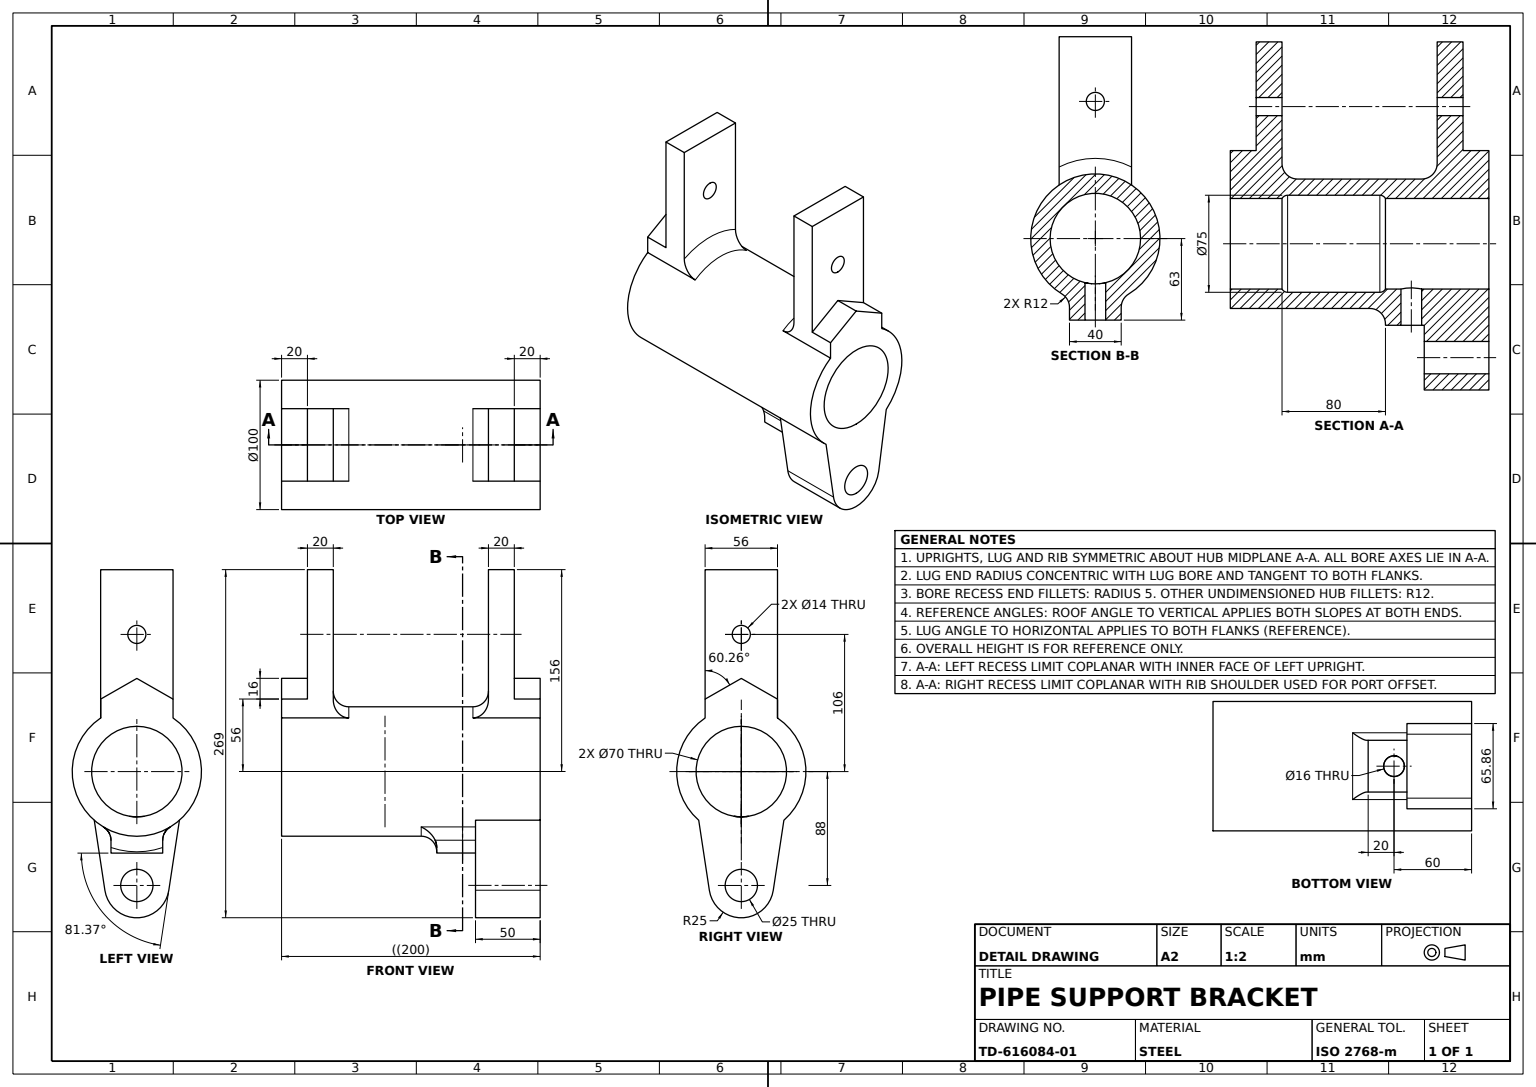
ISO-10303-21;
HEADER;
FILE_DESCRIPTION((''),'2;1');
FILE_NAME('','',(''),(''),'','','');
FILE_SCHEMA(('AUTOMOTIVE_DESIGN'));
ENDSEC;
DATA;
#1=APPLICATION_CONTEXT('');
#2=PRODUCT_CONTEXT('',#1,'mechanical');
#3=PRODUCT('','','',(#2));
#4=PRODUCT_DEFINITION_FORMATION('','',#3);
#5=PRODUCT_DEFINITION_CONTEXT('',#1,'design');
#6=PRODUCT_DEFINITION('','',#4,#5);
#7=PRODUCT_DEFINITION_SHAPE('','',#6);
#8=(LENGTH_UNIT()NAMED_UNIT(*)SI_UNIT(.MILLI.,.METRE.));
#9=(NAMED_UNIT(*)PLANE_ANGLE_UNIT()SI_UNIT($,.RADIAN.));
#10=(NAMED_UNIT(*)SI_UNIT($,.STERADIAN.)SOLID_ANGLE_UNIT());
#11=UNCERTAINTY_MEASURE_WITH_UNIT(LENGTH_MEASURE(0.005),#8,'distance_accuracy_value','');
#12=(GEOMETRIC_REPRESENTATION_CONTEXT(3)GLOBAL_UNCERTAINTY_ASSIGNED_CONTEXT((#11))GLOBAL_UNIT_ASSIGNED_CONTEXT((#8,#9,#10))REPRESENTATION_CONTEXT('',''));
#13=CARTESIAN_POINT('',(-28.,-80.,156.));
#14=VERTEX_POINT('',#13);
#15=CARTESIAN_POINT('',(28.,-80.,156.));
#16=VERTEX_POINT('',#15);
#17=DIRECTION('',(1.,0.,0.));
#18=VECTOR('',#17,1000.);
#19=LINE('',#13,#18);
#20=EDGE_CURVE('',#14,#16,#19,.T.);
#21=ORIENTED_EDGE('',*,*,#20,.T.);
#22=CARTESIAN_POINT('',(28.,-60.,156.));
#23=VERTEX_POINT('',#22);
#24=DIRECTION('',(0.,-1.,0.));
#25=VECTOR('',#24,1000.);
#26=LINE('',#22,#25);
#27=EDGE_CURVE('',#23,#16,#26,.T.);
#28=ORIENTED_EDGE('',*,*,#27,.F.);
#29=CARTESIAN_POINT('',(-28.,-60.,156.));
#30=VERTEX_POINT('',#29);
#31=LINE('',#29,#18);
#32=EDGE_CURVE('',#30,#23,#31,.T.);
#33=ORIENTED_EDGE('',*,*,#32,.F.);
#34=LINE('',#29,#25);
#35=EDGE_CURVE('',#30,#14,#34,.T.);
#36=ORIENTED_EDGE('',*,*,#35,.T.);
#37=EDGE_LOOP('',(#21,#28,#33,#36));
#38=FACE_BOUND('',#37,.T.);
#39=DIRECTION('',(0.,0.,-1.));
#40=DIRECTION('',(-1.,0.,0.));
#41=AXIS2_PLACEMENT_3D('',#29,#39,#40);
#42=PLANE('',#41);
#43=ADVANCED_FACE('',(#38),#42,.F.);
#44=CARTESIAN_POINT('',(0.,-80.,113.));
#45=VERTEX_POINT('',#44);
#46=CARTESIAN_POINT('',(0.,-80.,106.));
#47=DIRECTION('',(0.,1.,0.));
#48=DIRECTION('',(0.,0.,1.));
#49=AXIS2_PLACEMENT_3D('',#46,#47,#48);
#50=CIRCLE('',#49,7.);
#51=EDGE_CURVE('',#45,#45,#50,.T.);
#52=ORIENTED_EDGE('',*,*,#51,.F.);
#53=EDGE_LOOP('',(#52));
#54=FACE_BOUND('',#53,.T.);
#55=CARTESIAN_POINT('',(0.,-60.,113.));
#56=VERTEX_POINT('',#55);
#57=CARTESIAN_POINT('',(0.,-60.,106.));
#58=AXIS2_PLACEMENT_3D('',#57,#47,#48);
#59=CIRCLE('',#58,7.);
#60=EDGE_CURVE('',#56,#56,#59,.T.);
#61=ORIENTED_EDGE('',*,*,#60,.T.);
#62=EDGE_LOOP('',(#61));
#63=FACE_BOUND('',#62,.T.);
#64=CARTESIAN_POINT('',(0.,80.,106.));
#65=AXIS2_PLACEMENT_3D('',#64,#24,#39);
#66=CYLINDRICAL_SURFACE('',#65,7.);
#67=ADVANCED_FACE('',(#54,#63),#66,.F.);
#68=CARTESIAN_POINT('',(0.,-55.669873,-37.5));
#69=VERTEX_POINT('',#68);
#70=CARTESIAN_POINT('',(0.,-55.669873,0.));
#71=AXIS2_PLACEMENT_3D('',#70,#24,#39);
#72=CIRCLE('',#71,37.5);
#73=EDGE_CURVE('',#69,#69,#72,.F.);
#74=ORIENTED_EDGE('',*,*,#73,.T.);
#75=EDGE_LOOP('',(#74));
#76=FACE_BOUND('',#75,.T.);
#77=CARTESIAN_POINT('',(0.,-60.,-35.));
#78=VERTEX_POINT('',#77);
#79=CARTESIAN_POINT('',(0.,-60.,0.));
#80=AXIS2_PLACEMENT_3D('',#79,#24,#39);
#81=CIRCLE('',#80,35.);
#82=EDGE_CURVE('',#78,#78,#81,.F.);
#83=ORIENTED_EDGE('',*,*,#82,.F.);
#84=EDGE_LOOP('',(#83));
#85=FACE_BOUND('',#84,.T.);
#86=TOROIDAL_SURFACE('',#71,32.5,5.);
#87=ADVANCED_FACE('',(#76,#85),#86,.F.);
#88=CARTESIAN_POINT('',(0.,20.,-35.));
#89=VERTEX_POINT('',#88);
#90=CARTESIAN_POINT('',(0.,20.,0.));
#91=AXIS2_PLACEMENT_3D('',#90,#24,#39);
#92=CIRCLE('',#91,35.);
#93=EDGE_CURVE('',#89,#89,#92,.F.);
#94=ORIENTED_EDGE('',*,*,#93,.F.);
#95=EDGE_LOOP('',(#94));
#96=FACE_BOUND('',#95,.T.);
#97=CARTESIAN_POINT('',(8.,40.,-34.07345));
#98=VERTEX_POINT('',#97);
#99=CARTESIAN_POINT('',(7.575345,43.162099,-34.177167));
#100=CARTESIAN_POINT('',(8.211573,39.997592,-34.021762));
#101=CARTESIAN_POINT('',(7.578363,36.847533,-34.176486));
#102=CARTESIAN_POINT('',(5.801674,34.196418,-34.54076));
#103=CARTESIAN_POINT('',(3.152048,32.421651,-34.900124));
#104=CARTESIAN_POINT('',(0.005682,31.79015,-35.049729));
#105=CARTESIAN_POINT('',(-3.145527,32.417757,-34.900958));
#106=CARTESIAN_POINT('',(-5.803296,34.197129,-34.540575));
#107=CARTESIAN_POINT('',(-7.579059,36.849247,-34.176286));
#108=CARTESIAN_POINT('',(-8.20982,39.996413,-34.022177));
#109=CARTESIAN_POINT('',(-7.581658,43.144978,-34.175707));
#110=CARTESIAN_POINT('',(-5.807641,45.797608,-34.539704));
#111=CARTESIAN_POINT('',(-3.157808,47.576789,-34.899734));
#112=CARTESIAN_POINT('',(-0.004516,48.210487,-35.049891));
#113=CARTESIAN_POINT('',(3.146995,47.581253,-34.9007));
#114=CARTESIAN_POINT('',(5.799133,45.805003,-34.541192));
#115=B_SPLINE_CURVE_WITH_KNOTS('',3,(#99,#100,#101,#102,#103,#104,#105,#106,#107,#108,#109,#110,#111,#112,#113,#114,#99,#100,#101),.UNSPECIFIED.,.T.,.F.,(1,1,1,1,1,1,1,1,1,1,1,1,1,1,1,1,1,1,1,1,1,1,1),(-0.009409243,-0.006272829,-0.003136414,0.,0.003136414,0.006272829,0.009409243,0.012545657,0.015682072,0.018818486,0.0219549,0.025091314,0.028227729,0.031364143,0.034500557,0.037636972,0.040773386,0.0439098,0.047046215,0.050182629,0.053319043,0.056455457,0.059591872),.UNSPECIFIED.);
#116=EDGE_CURVE('',#98,#98,#115,.T.);
#117=ORIENTED_EDGE('',*,*,#116,.T.);
#118=EDGE_LOOP('',(#117));
#119=FACE_BOUND('',#118,.T.);
#120=CARTESIAN_POINT('',(0.,100.,-35.));
#121=VERTEX_POINT('',#120);
#122=CARTESIAN_POINT('',(0.,100.,0.));
#123=AXIS2_PLACEMENT_3D('',#122,#24,#39);
#124=CIRCLE('',#123,35.);
#125=EDGE_CURVE('',#121,#121,#124,.T.);
#126=ORIENTED_EDGE('',*,*,#125,.F.);
#127=EDGE_LOOP('',(#126));
#128=FACE_BOUND('',#127,.T.);
#129=CARTESIAN_POINT('',(0.,-100.,0.));
#130=AXIS2_PLACEMENT_3D('',#129,#47,#48);
#131=CYLINDRICAL_SURFACE('',#130,35.);
#132=ADVANCED_FACE('',(#96,#119,#128),#131,.F.);
#133=CARTESIAN_POINT('',(-28.,60.,156.));
#134=VERTEX_POINT('',#133);
#135=CARTESIAN_POINT('',(-28.,80.,156.));
#136=VERTEX_POINT('',#135);
#137=VECTOR('',#47,1000.);
#138=LINE('',#133,#137);
#139=EDGE_CURVE('',#134,#136,#138,.T.);
#140=ORIENTED_EDGE('',*,*,#139,.F.);
#141=CARTESIAN_POINT('',(28.,60.,156.));
#142=VERTEX_POINT('',#141);
#143=LINE('',#133,#18);
#144=EDGE_CURVE('',#134,#142,#143,.T.);
#145=ORIENTED_EDGE('',*,*,#144,.T.);
#146=CARTESIAN_POINT('',(28.,80.,156.));
#147=VERTEX_POINT('',#146);
#148=LINE('',#141,#137);
#149=EDGE_CURVE('',#142,#147,#148,.T.);
#150=ORIENTED_EDGE('',*,*,#149,.T.);
#151=LINE('',#135,#18);
#152=EDGE_CURVE('',#136,#147,#151,.T.);
#153=ORIENTED_EDGE('',*,*,#152,.F.);
#154=EDGE_LOOP('',(#140,#145,#150,#153));
#155=FACE_BOUND('',#154,.T.);
#156=AXIS2_PLACEMENT_3D('',#133,#48,#17);
#157=PLANE('',#156);
#158=ADVANCED_FACE('',(#155),#157,.T.);
#159=CARTESIAN_POINT('',(0.,60.,113.));
#160=VERTEX_POINT('',#159);
#161=CARTESIAN_POINT('',(0.,60.,106.));
#162=AXIS2_PLACEMENT_3D('',#161,#47,#48);
#163=CIRCLE('',#162,7.);
#164=EDGE_CURVE('',#160,#160,#163,.T.);
#165=ORIENTED_EDGE('',*,*,#164,.F.);
#166=EDGE_LOOP('',(#165));
#167=FACE_BOUND('',#166,.T.);
#168=CARTESIAN_POINT('',(0.,80.,99.));
#169=VERTEX_POINT('',#168);
#170=CIRCLE('',#65,7.);
#171=EDGE_CURVE('',#169,#169,#170,.T.);
#172=ORIENTED_EDGE('',*,*,#171,.F.);
#173=EDGE_LOOP('',(#172));
#174=FACE_BOUND('',#173,.T.);
#175=ADVANCED_FACE('',(#167,#174),#66,.F.);
#176=CARTESIAN_POINT('',(0.,15.669873,37.5));
#177=VERTEX_POINT('',#176);
#178=CARTESIAN_POINT('',(0.,15.669873,0.));
#179=AXIS2_PLACEMENT_3D('',#178,#47,#48);
#180=CIRCLE('',#179,37.5);
#181=EDGE_CURVE('',#177,#177,#180,.T.);
#182=ORIENTED_EDGE('',*,*,#181,.F.);
#183=EDGE_LOOP('',(#182));
#184=FACE_BOUND('',#183,.T.);
#185=ORIENTED_EDGE('',*,*,#93,.T.);
#186=EDGE_LOOP('',(#185));
#187=FACE_BOUND('',#186,.T.);
#188=TOROIDAL_SURFACE('',#179,32.5,5.);
#189=ADVANCED_FACE('',(#184,#187),#188,.F.);
#190=CARTESIAN_POINT('',(-20.,50.,-53.103672));
#191=VERTEX_POINT('',#190);
#192=CARTESIAN_POINT('',(-25.806452,50.,-42.825542));
#193=VERTEX_POINT('',#192);
#194=CARTESIAN_POINT('',(-32.,50.,-53.103672));
#195=AXIS2_PLACEMENT_3D('',#194,#24,#39);
#196=CIRCLE('',#195,12.);
#197=EDGE_CURVE('',#191,#193,#196,.T.);
#198=ORIENTED_EDGE('',*,*,#197,.T.);
#199=CARTESIAN_POINT('',(-32.93242,50.,-37.622543));
#200=VERTEX_POINT('',#199);
#201=CARTESIAN_POINT('',(0.,50.,0.));
#202=AXIS2_PLACEMENT_3D('',#201,#24,#39);
#203=CIRCLE('',#202,50.);
#204=EDGE_CURVE('',#200,#193,#203,.T.);
#205=ORIENTED_EDGE('',*,*,#204,.F.);
#206=CARTESIAN_POINT('',(-24.71693,50.,-91.751446));
#207=VERTEX_POINT('',#206);
#208=CARTESIAN_POINT('',(-35.,50.,-24.));
#209=DIRECTION('',(0.150057853,0.,-0.988677218));
#210=VECTOR('',#209,1000.);
#211=LINE('',#208,#210);
#212=EDGE_CURVE('',#200,#207,#211,.T.);
#213=ORIENTED_EDGE('',*,*,#212,.T.);
#214=CARTESIAN_POINT('',(24.71693,50.,-91.751446));
#215=VERTEX_POINT('',#214);
#216=CARTESIAN_POINT('',(0.,50.,-88.));
#217=AXIS2_PLACEMENT_3D('',#216,#24,#17);
#218=CIRCLE('',#217,25.);
#219=EDGE_CURVE('',#207,#215,#218,.T.);
#220=ORIENTED_EDGE('',*,*,#219,.T.);
#221=CARTESIAN_POINT('',(32.93242,50.,-37.622543));
#222=VERTEX_POINT('',#221);
#223=DIRECTION('',(0.150057853,0.,0.988677218));
#224=VECTOR('',#223,1000.);
#225=LINE('',#214,#224);
#226=EDGE_CURVE('',#215,#222,#225,.T.);
#227=ORIENTED_EDGE('',*,*,#226,.T.);
#228=CARTESIAN_POINT('',(25.806452,50.,-42.825542));
#229=VERTEX_POINT('',#228);
#230=EDGE_CURVE('',#229,#222,#203,.T.);
#231=ORIENTED_EDGE('',*,*,#230,.F.);
#232=CARTESIAN_POINT('',(20.,50.,-53.103672));
#233=VERTEX_POINT('',#232);
#234=CARTESIAN_POINT('',(32.,50.,-53.103672));
#235=AXIS2_PLACEMENT_3D('',#234,#24,#39);
#236=CIRCLE('',#235,12.);
#237=EDGE_CURVE('',#229,#233,#236,.T.);
#238=ORIENTED_EDGE('',*,*,#237,.T.);
#239=CARTESIAN_POINT('',(20.,50.,-63.));
#240=VERTEX_POINT('',#239);
#241=VECTOR('',#48,1000.);
#242=LINE('',#239,#241);
#243=EDGE_CURVE('',#240,#233,#242,.T.);
#244=ORIENTED_EDGE('',*,*,#243,.F.);
#245=CARTESIAN_POINT('',(-20.,50.,-63.));
#246=VERTEX_POINT('',#245);
#247=LINE('',#245,#18);
#248=EDGE_CURVE('',#246,#240,#247,.T.);
#249=ORIENTED_EDGE('',*,*,#248,.F.);
#250=CARTESIAN_POINT('',(-20.,50.,-36.75));
#251=VECTOR('',#39,1000.);
#252=LINE('',#250,#251);
#253=EDGE_CURVE('',#191,#246,#252,.T.);
#254=ORIENTED_EDGE('',*,*,#253,.F.);
#255=EDGE_LOOP('',(#198,#205,#213,#220,#227,#231,#238,#244,#249,#254));
#256=FACE_BOUND('',#255,.T.);
#257=CARTESIAN_POINT('',(0.,50.,-75.5));
#258=VERTEX_POINT('',#257);
#259=AXIS2_PLACEMENT_3D('',#216,#47,#48);
#260=CIRCLE('',#259,12.5);
#261=EDGE_CURVE('',#258,#258,#260,.T.);
#262=ORIENTED_EDGE('',*,*,#261,.T.);
#263=EDGE_LOOP('',(#262));
#264=FACE_BOUND('',#263,.T.);
#265=AXIS2_PLACEMENT_3D('',#216,#24,#39);
#266=PLANE('',#265);
#267=ADVANCED_FACE('',(#256,#264),#266,.T.);
#268=CARTESIAN_POINT('',(-28.,-100.,41.42463));
#269=VERTEX_POINT('',#268);
#270=CARTESIAN_POINT('',(28.,-100.,41.42463));
#271=VERTEX_POINT('',#270);
#272=AXIS2_PLACEMENT_3D('',#129,#24,#17);
#273=CIRCLE('',#272,50.);
#274=EDGE_CURVE('',#269,#271,#273,.T.);
#275=ORIENTED_EDGE('',*,*,#274,.T.);
#276=CARTESIAN_POINT('',(28.,-100.,56.));
#277=VERTEX_POINT('',#276);
#278=LINE('',#270,#241);
#279=EDGE_CURVE('',#271,#277,#278,.T.);
#280=ORIENTED_EDGE('',*,*,#279,.T.);
#281=CARTESIAN_POINT('',(0.,-100.,72.));
#282=VERTEX_POINT('',#281);
#283=DIRECTION('',(-0.868243142,0.,0.496138938));
#284=VECTOR('',#283,1000.);
#285=LINE('',#276,#284);
#286=EDGE_CURVE('',#277,#282,#285,.T.);
#287=ORIENTED_EDGE('',*,*,#286,.T.);
#288=CARTESIAN_POINT('',(-28.,-100.,56.));
#289=VERTEX_POINT('',#288);
#290=DIRECTION('',(-0.868243142,0.,-0.496138938));
#291=VECTOR('',#290,1000.);
#292=LINE('',#281,#291);
#293=EDGE_CURVE('',#282,#289,#292,.T.);
#294=ORIENTED_EDGE('',*,*,#293,.T.);
#295=LINE('',#288,#251);
#296=EDGE_CURVE('',#289,#269,#295,.T.);
#297=ORIENTED_EDGE('',*,*,#296,.T.);
#298=EDGE_LOOP('',(#275,#280,#287,#294,#297));
#299=FACE_BOUND('',#298,.T.);
#300=CARTESIAN_POINT('',(0.,-100.,35.));
#301=VERTEX_POINT('',#300);
#302=CIRCLE('',#130,35.);
#303=EDGE_CURVE('',#301,#301,#302,.T.);
#304=ORIENTED_EDGE('',*,*,#303,.T.);
#305=EDGE_LOOP('',(#304));
#306=FACE_BOUND('',#305,.T.);
#307=AXIS2_PLACEMENT_3D('',#129,#24,#39);
#308=PLANE('',#307);
#309=ADVANCED_FACE('',(#299,#306),#308,.T.);
#310=ORIENTED_EDGE('',*,*,#279,.F.);
#311=CARTESIAN_POINT('',(28.,-48.,41.42463));
#312=VERTEX_POINT('',#311);
#313=CARTESIAN_POINT('',(28.,-80.,41.42463));
#314=LINE('',#313,#25);
#315=EDGE_CURVE('',#312,#271,#314,.T.);
#316=ORIENTED_EDGE('',*,*,#315,.F.);
#317=CARTESIAN_POINT('',(28.,-60.,55.317267));
#318=VERTEX_POINT('',#317);
#319=CARTESIAN_POINT('',(28.,-48.855069,41.42463));
#320=CARTESIAN_POINT('',(28.,-50.526578,41.641141));
#321=CARTESIAN_POINT('',(28.,-53.719044,42.897489));
#322=CARTESIAN_POINT('',(28.,-56.979853,45.714878));
#323=CARTESIAN_POINT('',(28.,-59.431487,50.256632));
#324=CARTESIAN_POINT('',(28.,-60.,53.612888));
#325=B_SPLINE_CURVE_WITH_KNOTS('',3,(#311,#319,#320,#321,#322,#323,#324,#317),.UNSPECIFIED.,.F.,.F.,(4,1,1,1,1,4),(0.,0.002524701,0.005049402,0.010098805,0.015148207,0.02019761),.UNSPECIFIED.);
#326=EDGE_CURVE('',#312,#318,#325,.T.);
#327=ORIENTED_EDGE('',*,*,#326,.T.);
#328=LINE('',#22,#251);
#329=EDGE_CURVE('',#23,#318,#328,.T.);
#330=ORIENTED_EDGE('',*,*,#329,.F.);
#331=ORIENTED_EDGE('',*,*,#27,.T.);
#332=CARTESIAN_POINT('',(28.,-80.,56.));
#333=VERTEX_POINT('',#332);
#334=LINE('',#15,#251);
#335=EDGE_CURVE('',#16,#333,#334,.T.);
#336=ORIENTED_EDGE('',*,*,#335,.T.);
#337=LINE('',#332,#25);
#338=EDGE_CURVE('',#333,#277,#337,.T.);
#339=ORIENTED_EDGE('',*,*,#338,.T.);
#340=EDGE_LOOP('',(#310,#316,#327,#330,#331,#336,#339));
#341=FACE_BOUND('',#340,.T.);
#342=AXIS2_PLACEMENT_3D('',#313,#17,#39);
#343=PLANE('',#342);
#344=ADVANCED_FACE('',(#341),#343,.T.);
#345=CARTESIAN_POINT('',(24.71693,100.,-91.751446));
#346=VERTEX_POINT('',#345);
#347=LINE('',#345,#25);
#348=EDGE_CURVE('',#346,#215,#347,.T.);
#349=ORIENTED_EDGE('',*,*,#348,.T.);
#350=ORIENTED_EDGE('',*,*,#219,.F.);
#351=CARTESIAN_POINT('',(-24.71693,100.,-91.751446));
#352=VERTEX_POINT('',#351);
#353=LINE('',#351,#25);
#354=EDGE_CURVE('',#352,#207,#353,.T.);
#355=ORIENTED_EDGE('',*,*,#354,.F.);
#356=CARTESIAN_POINT('',(0.,100.,-88.));
#357=AXIS2_PLACEMENT_3D('',#356,#24,#17);
#358=CIRCLE('',#357,25.);
#359=EDGE_CURVE('',#352,#346,#358,.T.);
#360=ORIENTED_EDGE('',*,*,#359,.T.);
#361=EDGE_LOOP('',(#349,#350,#355,#360));
#362=FACE_BOUND('',#361,.T.);
#363=AXIS2_PLACEMENT_3D('',#356,#24,#39);
#364=CYLINDRICAL_SURFACE('',#363,25.);
#365=ADVANCED_FACE('',(#362),#364,.T.);
#366=ORIENTED_EDGE('',*,*,#303,.F.);
#367=EDGE_LOOP('',(#366));
#368=FACE_BOUND('',#367,.T.);
#369=ORIENTED_EDGE('',*,*,#82,.T.);
#370=EDGE_LOOP('',(#369));
#371=FACE_BOUND('',#370,.T.);
#372=ADVANCED_FACE('',(#368,#371),#131,.F.);
#373=ORIENTED_EDGE('',*,*,#32,.T.);
#374=ORIENTED_EDGE('',*,*,#329,.T.);
#375=CARTESIAN_POINT('',(-28.,-60.,55.317267));
#376=VERTEX_POINT('',#375);
#377=AXIS2_PLACEMENT_3D('',#79,#47,#48);
#378=CIRCLE('',#377,62.);
#379=EDGE_CURVE('',#318,#376,#378,.F.);
#380=ORIENTED_EDGE('',*,*,#379,.T.);
#381=CARTESIAN_POINT('',(-28.,-60.,40.));
#382=LINE('',#381,#241);
#383=EDGE_CURVE('',#376,#30,#382,.T.);
#384=ORIENTED_EDGE('',*,*,#383,.T.);
#385=EDGE_LOOP('',(#373,#374,#380,#384));
#386=FACE_BOUND('',#385,.T.);
#387=ORIENTED_EDGE('',*,*,#60,.F.);
#388=EDGE_LOOP('',(#387));
#389=FACE_BOUND('',#388,.T.);
#390=PLANE('',#377);
#391=ADVANCED_FACE('',(#386,#389),#390,.T.);
#392=CARTESIAN_POINT('',(0.,80.,72.));
#393=VERTEX_POINT('',#392);
#394=CARTESIAN_POINT('',(0.,100.,72.));
#395=VERTEX_POINT('',#394);
#396=LINE('',#392,#137);
#397=EDGE_CURVE('',#393,#395,#396,.T.);
#398=ORIENTED_EDGE('',*,*,#397,.F.);
#399=CARTESIAN_POINT('',(28.,80.,56.));
#400=VERTEX_POINT('',#399);
#401=LINE('',#399,#284);
#402=EDGE_CURVE('',#400,#393,#401,.T.);
#403=ORIENTED_EDGE('',*,*,#402,.F.);
#404=CARTESIAN_POINT('',(28.,100.,56.));
#405=VERTEX_POINT('',#404);
#406=LINE('',#399,#137);
#407=EDGE_CURVE('',#400,#405,#406,.T.);
#408=ORIENTED_EDGE('',*,*,#407,.T.);
#409=LINE('',#404,#284);
#410=EDGE_CURVE('',#405,#395,#409,.T.);
#411=ORIENTED_EDGE('',*,*,#410,.T.);
#412=EDGE_LOOP('',(#398,#403,#408,#411));
#413=FACE_BOUND('',#412,.T.);
#414=DIRECTION('',(-0.496138938,0.,-0.868243142));
#415=AXIS2_PLACEMENT_3D('',#399,#414,#283);
#416=PLANE('',#415);
#417=ADVANCED_FACE('',(#413),#416,.F.);
#418=CARTESIAN_POINT('',(0.,-80.,72.));
#419=VERTEX_POINT('',#418);
#420=CARTESIAN_POINT('',(-28.,-80.,56.));
#421=VERTEX_POINT('',#420);
#422=LINE('',#418,#291);
#423=EDGE_CURVE('',#419,#421,#422,.T.);
#424=ORIENTED_EDGE('',*,*,#423,.T.);
#425=LINE('',#420,#25);
#426=EDGE_CURVE('',#421,#289,#425,.T.);
#427=ORIENTED_EDGE('',*,*,#426,.T.);
#428=ORIENTED_EDGE('',*,*,#293,.F.);
#429=LINE('',#418,#25);
#430=EDGE_CURVE('',#419,#282,#429,.T.);
#431=ORIENTED_EDGE('',*,*,#430,.F.);
#432=EDGE_LOOP('',(#424,#427,#428,#431));
#433=FACE_BOUND('',#432,.T.);
#434=DIRECTION('',(-0.496138938,0.,0.868243142));
#435=DIRECTION('',(0.868243142,0.,0.496138938));
#436=AXIS2_PLACEMENT_3D('',#418,#434,#435);
#437=PLANE('',#436);
#438=ADVANCED_FACE('',(#433),#437,.T.);
#439=CARTESIAN_POINT('',(-28.,60.,55.317267));
#440=VERTEX_POINT('',#439);
#441=CARTESIAN_POINT('',(-28.,60.,40.));
#442=LINE('',#441,#241);
#443=EDGE_CURVE('',#440,#134,#442,.T.);
#444=ORIENTED_EDGE('',*,*,#443,.T.);
#445=ORIENTED_EDGE('',*,*,#139,.T.);
#446=CARTESIAN_POINT('',(-28.,80.,56.));
#447=VERTEX_POINT('',#446);
#448=CARTESIAN_POINT('',(-28.,80.,40.));
#449=LINE('',#448,#241);
#450=EDGE_CURVE('',#447,#136,#449,.T.);
#451=ORIENTED_EDGE('',*,*,#450,.F.);
#452=CARTESIAN_POINT('',(-28.,100.,56.));
#453=VERTEX_POINT('',#452);
#454=LINE('',#446,#137);
#455=EDGE_CURVE('',#447,#453,#454,.T.);
#456=ORIENTED_EDGE('',*,*,#455,.T.);
#457=CARTESIAN_POINT('',(-28.,100.,41.42463));
#458=VERTEX_POINT('',#457);
#459=LINE('',#452,#251);
#460=EDGE_CURVE('',#453,#458,#459,.T.);
#461=ORIENTED_EDGE('',*,*,#460,.T.);
#462=CARTESIAN_POINT('',(-28.,48.,41.42463));
#463=VERTEX_POINT('',#462);
#464=CARTESIAN_POINT('',(-28.,80.,41.42463));
#465=LINE('',#464,#137);
#466=EDGE_CURVE('',#463,#458,#465,.T.);
#467=ORIENTED_EDGE('',*,*,#466,.F.);
#468=CARTESIAN_POINT('',(-28.,48.855069,41.42463));
#469=CARTESIAN_POINT('',(-28.,50.526578,41.641141));
#470=CARTESIAN_POINT('',(-28.,53.719044,42.897489));
#471=CARTESIAN_POINT('',(-28.,56.979853,45.714878));
#472=CARTESIAN_POINT('',(-28.,59.431487,50.256632));
#473=CARTESIAN_POINT('',(-28.,60.,53.612888));
#474=B_SPLINE_CURVE_WITH_KNOTS('',3,(#462,#468,#469,#470,#471,#472,#473,#439),.UNSPECIFIED.,.F.,.F.,(4,1,1,1,1,4),(0.,0.002524701,0.005049402,0.010098805,0.015148207,0.02019761),.UNSPECIFIED.);
#475=EDGE_CURVE('',#463,#440,#474,.T.);
#476=ORIENTED_EDGE('',*,*,#475,.T.);
#477=EDGE_LOOP('',(#444,#445,#451,#456,#461,#467,#476));
#478=FACE_BOUND('',#477,.T.);
#479=AXIS2_PLACEMENT_3D('',#446,#17,#39);
#480=PLANE('',#479);
#481=ADVANCED_FACE('',(#478),#480,.F.);
#482=ORIENTED_EDGE('',*,*,#212,.F.);
#483=CARTESIAN_POINT('',(-32.93242,100.,-37.622543));
#484=VERTEX_POINT('',#483);
#485=CARTESIAN_POINT('',(-32.93242,-100.,-37.622543));
#486=LINE('',#485,#137);
#487=EDGE_CURVE('',#484,#200,#486,.F.);
#488=ORIENTED_EDGE('',*,*,#487,.F.);
#489=CARTESIAN_POINT('',(-35.,100.,-24.));
#490=LINE('',#489,#210);
#491=EDGE_CURVE('',#484,#352,#490,.T.);
#492=ORIENTED_EDGE('',*,*,#491,.T.);
#493=ORIENTED_EDGE('',*,*,#354,.T.);
#494=EDGE_LOOP('',(#482,#488,#492,#493));
#495=FACE_BOUND('',#494,.T.);
#496=DIRECTION('',(-0.988677218,0.,-0.150057853));
#497=DIRECTION('',(-0.150057853,0.,0.988677218));
#498=AXIS2_PLACEMENT_3D('',#489,#496,#497);
#499=PLANE('',#498);
#500=ADVANCED_FACE('',(#495),#499,.T.);
#501=ORIENTED_EDGE('',*,*,#181,.T.);
#502=EDGE_LOOP('',(#501));
#503=FACE_BOUND('',#502,.T.);
#504=ORIENTED_EDGE('',*,*,#73,.F.);
#505=EDGE_LOOP('',(#504));
#506=FACE_BOUND('',#505,.T.);
#507=CYLINDRICAL_SURFACE('',#91,37.5);
#508=ADVANCED_FACE('',(#503,#506),#507,.F.);
#509=ORIENTED_EDGE('',*,*,#455,.F.);
#510=LINE('',#392,#291);
#511=EDGE_CURVE('',#393,#447,#510,.T.);
#512=ORIENTED_EDGE('',*,*,#511,.F.);
#513=ORIENTED_EDGE('',*,*,#397,.T.);
#514=LINE('',#394,#291);
#515=EDGE_CURVE('',#395,#453,#514,.T.);
#516=ORIENTED_EDGE('',*,*,#515,.T.);
#517=EDGE_LOOP('',(#509,#512,#513,#516));
#518=FACE_BOUND('',#517,.T.);
#519=DIRECTION('',(0.496138938,0.,-0.868243142));
#520=AXIS2_PLACEMENT_3D('',#392,#519,#290);
#521=PLANE('',#520);
#522=ADVANCED_FACE('',(#518),#521,.F.);
#523=CARTESIAN_POINT('',(25.806452,8.,-42.825542));
#524=VERTEX_POINT('',#523);
#525=CARTESIAN_POINT('',(25.806452,-100.,-42.825542));
#526=LINE('',#525,#137);
#527=EDGE_CURVE('',#524,#229,#526,.T.);
#528=ORIENTED_EDGE('',*,*,#527,.F.);
#529=CARTESIAN_POINT('',(20.,18.788208,-53.103672));
#530=VERTEX_POINT('',#529);
#531=CARTESIAN_POINT('',(20.,18.209958,-51.835147));
#532=CARTESIAN_POINT('',(20.289493,17.125512,-50.109405));
#533=CARTESIAN_POINT('',(21.062355,15.385214,-48.084215));
#534=CARTESIAN_POINT('',(22.506626,12.634479,-45.415839));
#535=CARTESIAN_POINT('',(24.240008,10.036539,-43.769473));
#536=B_SPLINE_CURVE_WITH_KNOTS('',3,(#529,#531,#532,#533,#534,#535,#523),.UNSPECIFIED.,.F.,.F.,(4,1,1,1,4),(0.,0.004105794,0.006158691,0.008211588,0.016423176),.UNSPECIFIED.);
#537=EDGE_CURVE('',#530,#524,#536,.T.);
#538=ORIENTED_EDGE('',*,*,#537,.F.);
#539=CARTESIAN_POINT('',(20.,20.,-53.103672));
#540=LINE('',#539,#25);
#541=EDGE_CURVE('',#233,#530,#540,.T.);
#542=ORIENTED_EDGE('',*,*,#541,.F.);
#543=ORIENTED_EDGE('',*,*,#237,.F.);
#544=EDGE_LOOP('',(#528,#538,#542,#543));
#545=FACE_BOUND('',#544,.T.);
#546=CARTESIAN_POINT('',(32.,-100.,-53.103672));
#547=AXIS2_PLACEMENT_3D('',#546,#47,#48);
#548=CYLINDRICAL_SURFACE('',#547,12.);
#549=ADVANCED_FACE('',(#545),#548,.F.);
#550=CARTESIAN_POINT('',(0.,100.,-100.5));
#551=VERTEX_POINT('',#550);
#552=CIRCLE('',#363,12.5);
#553=EDGE_CURVE('',#551,#551,#552,.T.);
#554=ORIENTED_EDGE('',*,*,#553,.T.);
#555=EDGE_LOOP('',(#554));
#556=FACE_BOUND('',#555,.T.);
#557=CARTESIAN_POINT('',(28.,100.,41.42463));
#558=VERTEX_POINT('',#557);
#559=LINE('',#557,#241);
#560=EDGE_CURVE('',#558,#405,#559,.T.);
#561=ORIENTED_EDGE('',*,*,#560,.F.);
#562=CARTESIAN_POINT('',(32.93242,100.,-37.622543));
#563=VERTEX_POINT('',#562);
#564=AXIS2_PLACEMENT_3D('',#122,#24,#17);
#565=CIRCLE('',#564,50.);
#566=EDGE_CURVE('',#563,#558,#565,.T.);
#567=ORIENTED_EDGE('',*,*,#566,.F.);
#568=LINE('',#345,#224);
#569=EDGE_CURVE('',#346,#563,#568,.T.);
#570=ORIENTED_EDGE('',*,*,#569,.F.);
#571=ORIENTED_EDGE('',*,*,#359,.F.);
#572=ORIENTED_EDGE('',*,*,#491,.F.);
#573=EDGE_CURVE('',#458,#484,#565,.T.);
#574=ORIENTED_EDGE('',*,*,#573,.F.);
#575=ORIENTED_EDGE('',*,*,#460,.F.);
#576=ORIENTED_EDGE('',*,*,#515,.F.);
#577=ORIENTED_EDGE('',*,*,#410,.F.);
#578=EDGE_LOOP('',(#561,#567,#570,#571,#572,#574,#575,#576,#577));
#579=FACE_BOUND('',#578,.T.);
#580=ORIENTED_EDGE('',*,*,#125,.T.);
#581=EDGE_LOOP('',(#580));
#582=FACE_BOUND('',#581,.T.);
#583=PLANE('',#123);
#584=ADVANCED_FACE('',(#556,#579,#582),#583,.F.);
#585=CARTESIAN_POINT('',(20.,20.,-58.685603));
#586=VERTEX_POINT('',#585);
#587=CARTESIAN_POINT('',(-20.,20.,-58.685603));
#588=VERTEX_POINT('',#587);
#589=CIRCLE('',#91,62.);
#590=EDGE_CURVE('',#586,#588,#589,.F.);
#591=ORIENTED_EDGE('',*,*,#590,.T.);
#592=CARTESIAN_POINT('',(-20.,20.,-63.));
#593=VERTEX_POINT('',#592);
#594=CARTESIAN_POINT('',(-20.,20.,-36.75));
#595=LINE('',#594,#251);
#596=EDGE_CURVE('',#588,#593,#595,.T.);
#597=ORIENTED_EDGE('',*,*,#596,.T.);
#598=CARTESIAN_POINT('',(20.,20.,-63.));
#599=VERTEX_POINT('',#598);
#600=LINE('',#592,#18);
#601=EDGE_CURVE('',#593,#599,#600,.T.);
#602=ORIENTED_EDGE('',*,*,#601,.T.);
#603=LINE('',#598,#241);
#604=EDGE_CURVE('',#599,#586,#603,.T.);
#605=ORIENTED_EDGE('',*,*,#604,.T.);
#606=EDGE_LOOP('',(#591,#597,#602,#605));
#607=FACE_BOUND('',#606,.T.);
#608=PLANE('',#91);
#609=ADVANCED_FACE('',(#607),#608,.T.);
#610=CARTESIAN_POINT('',(-28.,-48.,41.42463));
#611=VERTEX_POINT('',#610);
#612=CARTESIAN_POINT('',(-28.,-80.,41.42463));
#613=LINE('',#612,#25);
#614=EDGE_CURVE('',#611,#269,#613,.T.);
#615=ORIENTED_EDGE('',*,*,#614,.F.);
#616=CARTESIAN_POINT('',(0.,-48.,0.));
#617=AXIS2_PLACEMENT_3D('',#616,#47,#48);
#618=CIRCLE('',#617,50.);
#619=EDGE_CURVE('',#611,#312,#618,.T.);
#620=ORIENTED_EDGE('',*,*,#619,.T.);
#621=ORIENTED_EDGE('',*,*,#315,.T.);
#622=ORIENTED_EDGE('',*,*,#274,.F.);
#623=EDGE_LOOP('',(#615,#620,#621,#622));
#624=FACE_BOUND('',#623,.T.);
#625=ORIENTED_EDGE('',*,*,#466,.T.);
#626=ORIENTED_EDGE('',*,*,#573,.T.);
#627=ORIENTED_EDGE('',*,*,#487,.T.);
#628=ORIENTED_EDGE('',*,*,#204,.T.);
#629=CARTESIAN_POINT('',(-25.806452,8.,-42.825542));
#630=VERTEX_POINT('',#629);
#631=CARTESIAN_POINT('',(-25.806452,-100.,-42.825542));
#632=LINE('',#631,#137);
#633=EDGE_CURVE('',#193,#630,#632,.F.);
#634=ORIENTED_EDGE('',*,*,#633,.T.);
#635=CARTESIAN_POINT('',(0.,8.,0.));
#636=AXIS2_PLACEMENT_3D('',#635,#24,#39);
#637=CIRCLE('',#636,50.);
#638=EDGE_CURVE('',#630,#524,#637,.T.);
#639=ORIENTED_EDGE('',*,*,#638,.T.);
#640=ORIENTED_EDGE('',*,*,#527,.T.);
#641=ORIENTED_EDGE('',*,*,#230,.T.);
#642=CARTESIAN_POINT('',(32.93242,-100.,-37.622543));
#643=LINE('',#642,#137);
#644=EDGE_CURVE('',#222,#563,#643,.T.);
#645=ORIENTED_EDGE('',*,*,#644,.T.);
#646=ORIENTED_EDGE('',*,*,#566,.T.);
#647=CARTESIAN_POINT('',(28.,48.,41.42463));
#648=VERTEX_POINT('',#647);
#649=CARTESIAN_POINT('',(28.,80.,41.42463));
#650=LINE('',#649,#137);
#651=EDGE_CURVE('',#648,#558,#650,.T.);
#652=ORIENTED_EDGE('',*,*,#651,.F.);
#653=CARTESIAN_POINT('',(0.,48.,0.));
#654=AXIS2_PLACEMENT_3D('',#653,#47,#48);
#655=CIRCLE('',#654,50.);
#656=EDGE_CURVE('',#648,#463,#655,.F.);
#657=ORIENTED_EDGE('',*,*,#656,.T.);
#658=EDGE_LOOP('',(#625,#626,#627,#628,#634,#639,#640,#641,#645,#646,#652,#657));
#659=FACE_BOUND('',#658,.T.);
#660=CYLINDRICAL_SURFACE('',#130,50.);
#661=ADVANCED_FACE('',(#624,#659),#660,.T.);
#662=ORIENTED_EDGE('',*,*,#164,.T.);
#663=EDGE_LOOP('',(#662));
#664=FACE_BOUND('',#663,.T.);
#665=CARTESIAN_POINT('',(28.,60.,55.317267));
#666=VERTEX_POINT('',#665);
#667=LINE('',#141,#251);
#668=EDGE_CURVE('',#142,#666,#667,.T.);
#669=ORIENTED_EDGE('',*,*,#668,.F.);
#670=ORIENTED_EDGE('',*,*,#144,.F.);
#671=ORIENTED_EDGE('',*,*,#443,.F.);
#672=CARTESIAN_POINT('',(0.,60.,0.));
#673=AXIS2_PLACEMENT_3D('',#672,#47,#48);
#674=CIRCLE('',#673,62.);
#675=EDGE_CURVE('',#440,#666,#674,.T.);
#676=ORIENTED_EDGE('',*,*,#675,.T.);
#677=EDGE_LOOP('',(#669,#670,#671,#676));
#678=FACE_BOUND('',#677,.T.);
#679=PLANE('',#673);
#680=ADVANCED_FACE('',(#664,#678),#679,.F.);
#681=ORIENTED_EDGE('',*,*,#261,.F.);
#682=EDGE_LOOP('',(#681));
#683=FACE_BOUND('',#682,.T.);
#684=ORIENTED_EDGE('',*,*,#553,.F.);
#685=EDGE_LOOP('',(#684));
#686=FACE_BOUND('',#685,.T.);
#687=CYLINDRICAL_SURFACE('',#259,12.5);
#688=ADVANCED_FACE('',(#683,#686),#687,.F.);
#689=ORIENTED_EDGE('',*,*,#35,.F.);
#690=ORIENTED_EDGE('',*,*,#383,.F.);
#691=CARTESIAN_POINT('',(-28.,-60.,53.61085));
#692=CARTESIAN_POINT('',(-28.,-59.430898,50.257137));
#693=CARTESIAN_POINT('',(-28.,-56.985191,45.725679));
#694=CARTESIAN_POINT('',(-28.,-53.091243,42.346481));
#695=CARTESIAN_POINT('',(-28.,-49.714621,41.42463));
#696=B_SPLINE_CURVE_WITH_KNOTS('',3,(#375,#691,#692,#693,#694,#695,#610),.UNSPECIFIED.,.F.,.F.,(4,1,1,1,4),(0.,0.005046392,0.010092784,0.015139176,0.020185568),.UNSPECIFIED.);
#697=EDGE_CURVE('',#376,#611,#696,.T.);
#698=ORIENTED_EDGE('',*,*,#697,.T.);
#699=ORIENTED_EDGE('',*,*,#614,.T.);
#700=ORIENTED_EDGE('',*,*,#296,.F.);
#701=ORIENTED_EDGE('',*,*,#426,.F.);
#702=CARTESIAN_POINT('',(-28.,-80.,40.));
#703=LINE('',#702,#241);
#704=EDGE_CURVE('',#421,#14,#703,.T.);
#705=ORIENTED_EDGE('',*,*,#704,.T.);
#706=EDGE_LOOP('',(#689,#690,#698,#699,#700,#701,#705));
#707=FACE_BOUND('',#706,.T.);
#708=AXIS2_PLACEMENT_3D('',#420,#40,#48);
#709=PLANE('',#708);
#710=ADVANCED_FACE('',(#707),#709,.T.);
#711=ORIENTED_EDGE('',*,*,#619,.F.);
#712=ORIENTED_EDGE('',*,*,#697,.F.);
#713=ORIENTED_EDGE('',*,*,#379,.F.);
#714=ORIENTED_EDGE('',*,*,#326,.F.);
#715=EDGE_LOOP('',(#711,#712,#713,#714));
#716=FACE_BOUND('',#715,.T.);
#717=TOROIDAL_SURFACE('',#617,62.,12.);
#718=ADVANCED_FACE('',(#716),#717,.F.);
#719=CARTESIAN_POINT('',(8.,40.,-63.));
#720=VERTEX_POINT('',#719);
#721=CARTESIAN_POINT('',(0.,40.,-63.));
#722=AXIS2_PLACEMENT_3D('',#721,#48,#17);
#723=CIRCLE('',#722,8.);
#724=EDGE_CURVE('',#720,#720,#723,.T.);
#725=ORIENTED_EDGE('',*,*,#724,.F.);
#726=EDGE_LOOP('',(#725));
#727=FACE_BOUND('',#726,.T.);
#728=ORIENTED_EDGE('',*,*,#116,.F.);
#729=EDGE_LOOP('',(#728));
#730=FACE_BOUND('',#729,.T.);
#731=CYLINDRICAL_SURFACE('',#722,8.);
#732=ADVANCED_FACE('',(#727,#730),#731,.F.);
#733=ORIENTED_EDGE('',*,*,#51,.T.);
#734=EDGE_LOOP('',(#733));
#735=FACE_BOUND('',#734,.T.);
#736=ORIENTED_EDGE('',*,*,#20,.F.);
#737=ORIENTED_EDGE('',*,*,#704,.F.);
#738=ORIENTED_EDGE('',*,*,#423,.F.);
#739=LINE('',#332,#284);
#740=EDGE_CURVE('',#333,#419,#739,.T.);
#741=ORIENTED_EDGE('',*,*,#740,.F.);
#742=ORIENTED_EDGE('',*,*,#335,.F.);
#743=EDGE_LOOP('',(#736,#737,#738,#741,#742));
#744=FACE_BOUND('',#743,.T.);
#745=CARTESIAN_POINT('',(0.,-80.,0.));
#746=AXIS2_PLACEMENT_3D('',#745,#47,#48);
#747=PLANE('',#746);
#748=ADVANCED_FACE('',(#735,#744),#747,.F.);
#749=LINE('',#598,#137);
#750=EDGE_CURVE('',#599,#240,#749,.T.);
#751=ORIENTED_EDGE('',*,*,#750,.F.);
#752=ORIENTED_EDGE('',*,*,#601,.F.);
#753=LINE('',#592,#137);
#754=EDGE_CURVE('',#593,#246,#753,.T.);
#755=ORIENTED_EDGE('',*,*,#754,.T.);
#756=ORIENTED_EDGE('',*,*,#248,.T.);
#757=EDGE_LOOP('',(#751,#752,#755,#756));
#758=FACE_BOUND('',#757,.T.);
#759=ORIENTED_EDGE('',*,*,#724,.T.);
#760=EDGE_LOOP('',(#759));
#761=FACE_BOUND('',#760,.T.);
#762=AXIS2_PLACEMENT_3D('',#592,#48,#17);
#763=PLANE('',#762);
#764=ADVANCED_FACE('',(#758,#761),#763,.F.);
#765=CARTESIAN_POINT('',(-20.,18.788208,-53.103672));
#766=VERTEX_POINT('',#765);
#767=CARTESIAN_POINT('',(-20.,20.,-56.752236));
#768=CARTESIAN_POINT('',(-20.,19.590103,-54.862815));
#769=B_SPLINE_CURVE_WITH_KNOTS('',3,(#587,#767,#768,#765),.UNSPECIFIED.,.F.,.F.,(4,4),(0.,0.005717812),.UNSPECIFIED.);
#770=EDGE_CURVE('',#588,#766,#769,.T.);
#771=ORIENTED_EDGE('',*,*,#770,.T.);
#772=LINE('',#190,#25);
#773=EDGE_CURVE('',#766,#191,#772,.F.);
#774=ORIENTED_EDGE('',*,*,#773,.T.);
#775=ORIENTED_EDGE('',*,*,#253,.T.);
#776=ORIENTED_EDGE('',*,*,#754,.F.);
#777=ORIENTED_EDGE('',*,*,#596,.F.);
#778=EDGE_LOOP('',(#771,#774,#775,#776,#777));
#779=FACE_BOUND('',#778,.T.);
#780=AXIS2_PLACEMENT_3D('',#594,#17,#39);
#781=PLANE('',#780);
#782=ADVANCED_FACE('',(#779),#781,.F.);
#783=ORIENTED_EDGE('',*,*,#430,.T.);
#784=ORIENTED_EDGE('',*,*,#286,.F.);
#785=ORIENTED_EDGE('',*,*,#338,.F.);
#786=ORIENTED_EDGE('',*,*,#740,.T.);
#787=EDGE_LOOP('',(#783,#784,#785,#786));
#788=FACE_BOUND('',#787,.T.);
#789=DIRECTION('',(0.496138938,0.,0.868243142));
#790=DIRECTION('',(0.868243142,0.,-0.496138938));
#791=AXIS2_PLACEMENT_3D('',#332,#789,#790);
#792=PLANE('',#791);
#793=ADVANCED_FACE('',(#788),#792,.T.);
#794=ORIENTED_EDGE('',*,*,#644,.F.);
#795=ORIENTED_EDGE('',*,*,#226,.F.);
#796=ORIENTED_EDGE('',*,*,#348,.F.);
#797=ORIENTED_EDGE('',*,*,#569,.T.);
#798=EDGE_LOOP('',(#794,#795,#796,#797));
#799=FACE_BOUND('',#798,.T.);
#800=DIRECTION('',(0.988677218,0.,-0.150057853));
#801=DIRECTION('',(-0.150057853,0.,-0.988677218));
#802=AXIS2_PLACEMENT_3D('',#345,#800,#801);
#803=PLANE('',#802);
#804=ADVANCED_FACE('',(#799),#803,.T.);
#805=ORIENTED_EDGE('',*,*,#171,.T.);
#806=EDGE_LOOP('',(#805));
#807=FACE_BOUND('',#806,.T.);
#808=ORIENTED_EDGE('',*,*,#511,.T.);
#809=ORIENTED_EDGE('',*,*,#450,.T.);
#810=ORIENTED_EDGE('',*,*,#152,.T.);
#811=LINE('',#146,#251);
#812=EDGE_CURVE('',#147,#400,#811,.T.);
#813=ORIENTED_EDGE('',*,*,#812,.T.);
#814=ORIENTED_EDGE('',*,*,#402,.T.);
#815=EDGE_LOOP('',(#808,#809,#810,#813,#814));
#816=FACE_BOUND('',#815,.T.);
#817=CARTESIAN_POINT('',(0.,80.,0.));
#818=AXIS2_PLACEMENT_3D('',#817,#47,#48);
#819=PLANE('',#818);
#820=ADVANCED_FACE('',(#807,#816),#819,.T.);
#821=ORIENTED_EDGE('',*,*,#633,.F.);
#822=ORIENTED_EDGE('',*,*,#197,.F.);
#823=ORIENTED_EDGE('',*,*,#773,.F.);
#824=CARTESIAN_POINT('',(-20.,18.209958,-51.835147));
#825=CARTESIAN_POINT('',(-20.289493,17.125512,-50.109405));
#826=CARTESIAN_POINT('',(-21.062355,15.385214,-48.084215));
#827=CARTESIAN_POINT('',(-22.506626,12.634479,-45.415839));
#828=CARTESIAN_POINT('',(-24.240008,10.036539,-43.769473));
#829=B_SPLINE_CURVE_WITH_KNOTS('',3,(#765,#824,#825,#826,#827,#828,#629),.UNSPECIFIED.,.F.,.F.,(4,1,1,1,4),(0.,0.004105794,0.006158691,0.008211588,0.016423176),.UNSPECIFIED.);
#830=EDGE_CURVE('',#630,#766,#829,.F.);
#831=ORIENTED_EDGE('',*,*,#830,.F.);
#832=EDGE_LOOP('',(#821,#822,#823,#831));
#833=FACE_BOUND('',#832,.T.);
#834=CARTESIAN_POINT('',(-32.,-100.,-53.103672));
#835=AXIS2_PLACEMENT_3D('',#834,#47,#48);
#836=CYLINDRICAL_SURFACE('',#835,12.);
#837=ADVANCED_FACE('',(#833),#836,.F.);
#838=ORIENTED_EDGE('',*,*,#590,.F.);
#839=CARTESIAN_POINT('',(20.,19.590155,-54.862928));
#840=CARTESIAN_POINT('',(20.,20.,-56.752322));
#841=B_SPLINE_CURVE_WITH_KNOTS('',3,(#529,#839,#840,#585),.UNSPECIFIED.,.F.,.F.,(4,4),(0.,0.005717794),.UNSPECIFIED.);
#842=EDGE_CURVE('',#530,#586,#841,.T.);
#843=ORIENTED_EDGE('',*,*,#842,.F.);
#844=ORIENTED_EDGE('',*,*,#537,.T.);
#845=ORIENTED_EDGE('',*,*,#638,.F.);
#846=ORIENTED_EDGE('',*,*,#830,.T.);
#847=ORIENTED_EDGE('',*,*,#770,.F.);
#848=EDGE_LOOP('',(#838,#843,#844,#845,#846,#847));
#849=FACE_BOUND('',#848,.T.);
#850=TOROIDAL_SURFACE('',#636,62.,12.);
#851=ADVANCED_FACE('',(#849),#850,.F.);
#852=ORIENTED_EDGE('',*,*,#656,.F.);
#853=CARTESIAN_POINT('',(28.,60.,53.61085));
#854=CARTESIAN_POINT('',(28.,59.430898,50.257137));
#855=CARTESIAN_POINT('',(28.,56.985191,45.725679));
#856=CARTESIAN_POINT('',(28.,53.091243,42.346481));
#857=CARTESIAN_POINT('',(28.,49.714621,41.42463));
#858=B_SPLINE_CURVE_WITH_KNOTS('',3,(#665,#853,#854,#855,#856,#857,#647),.UNSPECIFIED.,.F.,.F.,(4,1,1,1,4),(0.,0.005046392,0.010092784,0.015139176,0.020185568),.UNSPECIFIED.);
#859=EDGE_CURVE('',#666,#648,#858,.T.);
#860=ORIENTED_EDGE('',*,*,#859,.F.);
#861=ORIENTED_EDGE('',*,*,#675,.F.);
#862=ORIENTED_EDGE('',*,*,#475,.F.);
#863=EDGE_LOOP('',(#852,#860,#861,#862));
#864=FACE_BOUND('',#863,.T.);
#865=TOROIDAL_SURFACE('',#654,62.,12.);
#866=ADVANCED_FACE('',(#864),#865,.F.);
#867=ORIENTED_EDGE('',*,*,#243,.T.);
#868=ORIENTED_EDGE('',*,*,#541,.T.);
#869=ORIENTED_EDGE('',*,*,#842,.T.);
#870=ORIENTED_EDGE('',*,*,#604,.F.);
#871=ORIENTED_EDGE('',*,*,#750,.T.);
#872=EDGE_LOOP('',(#867,#868,#869,#870,#871));
#873=FACE_BOUND('',#872,.T.);
#874=AXIS2_PLACEMENT_3D('',#598,#40,#48);
#875=PLANE('',#874);
#876=ADVANCED_FACE('',(#873),#875,.F.);
#877=ORIENTED_EDGE('',*,*,#149,.F.);
#878=ORIENTED_EDGE('',*,*,#668,.T.);
#879=ORIENTED_EDGE('',*,*,#859,.T.);
#880=ORIENTED_EDGE('',*,*,#651,.T.);
#881=ORIENTED_EDGE('',*,*,#560,.T.);
#882=ORIENTED_EDGE('',*,*,#407,.F.);
#883=ORIENTED_EDGE('',*,*,#812,.F.);
#884=EDGE_LOOP('',(#877,#878,#879,#880,#881,#882,#883));
#885=FACE_BOUND('',#884,.T.);
#886=AXIS2_PLACEMENT_3D('',#649,#40,#48);
#887=PLANE('',#886);
#888=ADVANCED_FACE('',(#885),#887,.F.);
#889=CLOSED_SHELL('',(#43,#67,#87,#132,#158,#175,#189,#267,#309,#344,#365,#372,#391,#417,#438,#481,#500,#508,#522,#549,#584,#609,#661,#680,#688,#710,#718,#732,#748,#764,#782,#793,#804,#820,#837,#851,#866,#876,#888));
#890=MANIFOLD_SOLID_BREP('',#889);
#891=ADVANCED_BREP_SHAPE_REPRESENTATION('',(#890),#12);
#892=SHAPE_DEFINITION_REPRESENTATION(#7,#891);
ENDSEC;
END-ISO-10303-21;
